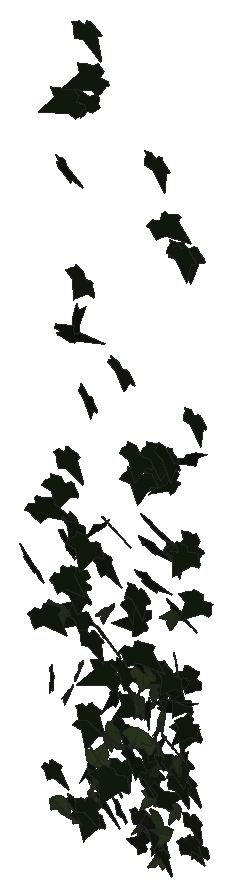
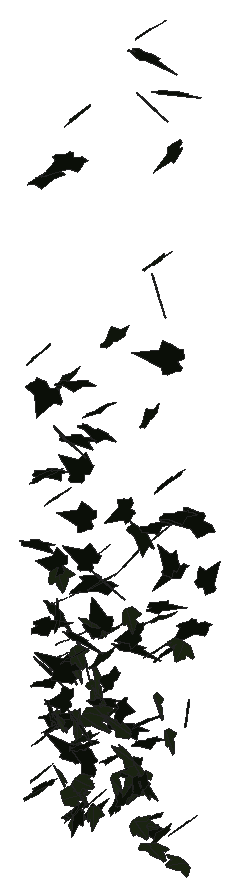
# SketchUp Ruby script. Lengths in inches.
U = 1.inch
M = Sketchup.active_model
def pt(a) = Geom::Point3d.new(a.map { |v| v * U })
def face(e, loops, mat)
  f = e.add_face(loops[0].map { |a| pt(a) })
  loops[1..].each { |l| e.add_face(l.map { |a| pt(a) }).erase! }
  f.material = f.back_material = mat if mat
  f
end
# faces: each face lists its corners as indices into pts; further lists are holes
def faces(e, pts, list, mat = nil) = list.each { |f| face(e, (f[0].is_a?(Array) ? f : [f]).map { |l| l.map { |i| pts[i] } }, mat) }
# xy, xz, yz: faces in a plane at the given z, y or x. An outline is a flat list of corners, or four numbers for a rectangle; further outlines are holes
def ring(l) = l.size == 4 ? [[l[0], l[1]], [l[2], l[1]], [l[2], l[3]], [l[0], l[3]]] : l.each_slice(2).to_a
def flat(e, list, mat, &to3) = list.each { |f| face(e, (f[0].is_a?(Array) ? f : [f]).map { |l| ring(l).map { |u, v| to3.(u, v) } }, mat) }
def xy(e, z, list, mat = nil) = flat(e, list, mat) { |x, y| [x, y, z] }
def xz(e, y, list, mat = nil) = flat(e, list, mat) { |x, z| [x, y, z] }
def yz(e, x, list, mat = nil) = flat(e, list, mat) { |y, z| [x, y, z] }
def lines(e, pts, list) = list.each { |a, b| e.add_line(pt(pts[a]), pt(pts[b])) }
# prism: a flat outline (further loops are holes) pulled along v
def prism(e, loops, v, mat = nil)
  f = face(e, loops, mat); d = Geom::Vector3d.new(v.map { |x| x * U })
  f.pushpull(f.normal.samedirection?(d) ? d.length : -d.length)
end
def box(e, o, s, mat = nil) = prism(e, [[o, [o[0] + s[0], o[1], o[2]], [o[0] + s[0], o[1] + s[1], o[2]], [o[0], o[1] + s[1], o[2]]]], [0, 0, s[2]], mat)
def at(x, y, z, deg = 0) = Geom::Transformation.translation(pt([x, y, z])) * Geom::Transformation.rotation(ORIGIN, Z_AXIS, deg.degrees)
def axes(o, x, y, z) = Geom::Transformation.new([*x, 0, *y, 0, *z, 0, *pt(o).to_a, 1])
def part(name) = M.definitions.add(name)
# library, detail: a bought-in or finely detailed component or shape, given as its bounding box
def library(name, o, s) = part(name).tap { |d| box(d.entities, o, s) }
def detail(e, o, s) = box(e.add_group.entities, o, s)
def put(e, d, t, mat = nil) = e.add_instance(d, t).tap { |i| i.material = mat if mat }
def group(e, t, mat = nil) = e.add_group.tap { |g| g.transformation = t; g.material = mat if mat }.entities
root = M.entities
M.materials.add("1026 AP 7946 SUNNY SIDE UP").color = [254, 231, 186]
M.materials.add("efeu1").color = [18, 25, 13]
M.materials.add("efeu2").color = [43, 57, 29]
c1 = part("ivyleaf_9")
p = [[1.54,2.16,1.25],[1.36,2.04,1.19],[-0.21,0.99,0.68],[-0.71,1.11,0.82],[-0.85,0.86,0.67],[-0.8,0.17,0.21],
  [-0.9,-0.01,0.1],[-0.67,-0.16,-0.02],[-0.08,-0.08,-0.05],[-0.03,-0.6,-0.4],[0.65,-0.88,-0.66],[0.83,-0.6,-0.49],
  [1.29,-0.42,-0.43],[1.8125,-0.07,-0.26],[1.21,0.44,0.15]]
faces(c1.entities,p,[[0,1,2,3,4,5,6,7,8,9,10,11,12,13,14]],"efeu1")
c2 = part("ivyleaf_10")
p = [[0,0.5,-0.03],[-0.0625,2.02,-0.43],[-0.19,2.01,-0.46],[-0.54,1.05,-0.29],[-0.52,0.625,-0.18],[-0.83,0.76,-0.28],
  [-1.16,0.64,-0.33],[-1.15,0.33,-0.24],[-0.77,-0.39,0.02],[-0.3,-0.51,0.16],[0.04,-0.48,0.23],[-0.02,2.01,-0.4375],
  [-0.06,2.01,-0.43],[0.04,-0.49,0.23],[0.67,-0.49,0.14],[1.38,0.36,-0.2],[1.375,0.51,-0.24],[0.81,0.65,-0.19],
  [0.62,0.59,-0.15],[0.6,1.09,-0.28],[0.5,1.23,-0.31]]
faces(c2.entities,p,[[0,1,2,3,4,5,6,7,8,9,10],[11,12,0,13,14,15,16,17,18,19,20]],"efeu2")
put(root,c1,axes([120.64,210.23,304.1],[0.28592,-0.32766,0.26056],[-0.14021,0.24083,0.38604],[-0.63741,-0.19995,0.03197]),"1026 AP 7946 SUNNY SIDE UP")
put(root,c1,axes([120.27,211.82,293.3125],[0.25007,-0.29162,-0.18402],[-0.05716,0.17966,-0.3376],[0.53333,0.156,0.0501]),"1026 AP 7946 SUNNY SIDE UP")
put(root,c2,axes([120.37,212.17,291.41],[-0.39726,-0.00522,-0.27921],[0.39286,-0.14811,-0.23789],[-0.16523,-0.3396,0.10568]),"1026 AP 7946 SUNNY SIDE UP")
put(root,c2,axes([120.76,211.63,301.71],[-0.60127,0.08137,-0.06025],[0.07732,-0.05071,-0.40105],[-0.13777,-0.38357,0.03786]),"1026 AP 7946 SUNNY SIDE UP")
put(root,c1,axes([120.63,211.45,298.32],[0.06531,-0.1363,-0.39031],[0.50627,-0.21622,0.11547],[-0.37825,-0.31294,0.08717]),"1026 AP 7946 SUNNY SIDE UP")
put(root,c2,axes([121.14,212.1,297.37],[0.09032,-0.38326,0.01758],[-0.00117,-0.01956,-0.39934],[0.6034,0.05733,-0.0034]),"1026 AP 7946 SUNNY SIDE UP")
put(root,c1,axes([120.64,210.47,307.37],[0.1737,-0.02062,-0.4547],[0.41121,0.36963,0.05181],[0.55979,-0.26512,0.10303]),"1026 AP 7946 SUNNY SIDE UP")
put(root,c1,axes([121.11,211.67,308.05],[-0.33308,-0.3602,-0.01481],[0.02704,0.00418,-0.43026],[0.56606,-0.21215,0.01184]),"1026 AP 7946 SUNNY SIDE UP")
put(root,c1,axes([120.99,210.36,302.12],[0.04492,-0.24383,-0.39442],[0.00693,0.38237,-0.2492],[0.71187,0.01167,0.02732]),"1026 AP 7946 SUNNY SIDE UP")
put(root,c1,axes([121.37,212.29,301.29],[-0.17419,-0.264,0.2771],[-0.14262,-0.25505,-0.29622],[0.57695,-0.14276,0.01044]),"1026 AP 7946 SUNNY SIDE UP")
put(root,c1,axes([121.31,211.56,309.73],[0.22359,-0.39067,-0.18284],[-0.06426,0.17145,-0.42686],[0.6702,0.14677,0.02007]),"1026 AP 7946 SUNNY SIDE UP")
put(root,c1,axes([120.99,211.83,315.69],[0.4611,-0.03933,0.35691],[0.54226,-0.03601,-0.30494],[0.08321,0.45264,0.00944]),"1026 AP 7946 SUNNY SIDE UP")
put(root,c1,axes([122.03,211.96,303.28],[-0.37134,-0.08589,0.31608],[-0.40952,-0.169,-0.25583],[0.28987,-0.34878,0.04348]),"1026 AP 7946 SUNNY SIDE UP")
put(root,c2,axes([121.82,212,298.82],[0.17687,-0.3738,-0.04632],[-0.03405,0.03821,-0.4018],[0.59064,0.11414,-0.00929]),"1026 AP 7946 SUNNY SIDE UP")
put(root,c1,axes([121.38,211.51,305.21],[0.11465,-0.13289,0.42396],[0.22216,-0.38793,-0.15682],[0.64387,0.15751,-0.02138]),"1026 AP 7946 SUNNY SIDE UP")
put(root,c1,axes([122.14,211.12,328.17],[-0.65585,-0.11577,0.19889],[-0.20333,-0.21101,-0.41799],[0.29082,-0.40862,0.15628]),"1026 AP 7946 SUNNY SIDE UP")
put(root,c1,axes([121.7,212.22,301.41],[-0.04768,-0.38202,0.08659],[0.00998,-0.08694,-0.39508],[0.61572,-0.02817,0.01311]),"1026 AP 7946 SUNNY SIDE UP")
put(root,c2,axes([122.04,212.1,291.61],[0.54998,0.07879,-0.16507],[-0.22999,-0.07736,-0.36756],[-0.16212,0.37706,-0.03853]),"1026 AP 7946 SUNNY SIDE UP")
put(root,c1,axes([121.8,211.83,302.75],[-0.15081,-0.36461,0.12107],[0.10561,-0.13732,-0.37662],[0.59406,-0.06815,0.09769]),"1026 AP 7946 SUNNY SIDE UP")
put(root,c1,axes([122.42,211.65,327.63],[0.03759,0.28344,0.38774],[-0.34589,0.33834,-0.24718],[-0.65288,-0.16293,0.15328]),"1026 AP 7946 SUNNY SIDE UP")
put(root,c1,axes([121.82,211.69,292.02],[0.07471,-0.33256,0.17753],[0.04916,-0.17149,-0.34702],[0.58827,0.05656,0.00645]),"1026 AP 7946 SUNNY SIDE UP")
put(root,c1,axes([121.91,210.5,325.17],[0.55052,-0.19879,-0.24116],[-0.25395,0.18079,-0.40792],[0.40915,0.3797,0.0713]),"1026 AP 7946 SUNNY SIDE UP")
put(root,c1,axes([122.21,211.28,306.54],[-0.11855,-0.3498,0.27052],[-0.07175,-0.26074,-0.37007],[0.6859,-0.08773,0.00804]),"1026 AP 7946 SUNNY SIDE UP")
put(root,c1,axes([122.07,212.21,312.61],[0.05601,-0.32266,0.29324],[0.03549,-0.28567,-0.33603],[0.67755,0.04164,-0.00664]),"1026 AP 7946 SUNNY SIDE UP")
put(root,c1,axes([122.15,210.25,304.42],[0.1826,-0.23016,-0.39573],[-0.15822,0.3719,-0.25961],[0.68431,0.1474,0.04557]),"1026 AP 7946 SUNNY SIDE UP")
put(root,c1,axes([122.17,211.89,331.63],[0.16087,-0.46178,-0.08563],[0.02278,0.08547,-0.48563],[0.7367,0.09819,0.03372]),"1026 AP 7946 SUNNY SIDE UP")
put(root,c2,axes([122.82,212.02,292.36],[-0.13485,-0.08859,0.3881],[-0.12572,-0.374,-0.11139],[0.59618,-0.0989,0.06429]),"1026 AP 7946 SUNNY SIDE UP")
put(root,c1,axes([122.76,211.85,294.38],[-0.41219,0.13402,-0.25345],[0.28629,-0.17592,-0.29869],[-0.3362,-0.31412,0.05639]),"1026 AP 7946 SUNNY SIDE UP")
put(root,c2,axes([122.8,212.14,292.47],[-0.14475,-0.32546,0.16154],[-0.06372,-0.15341,-0.34933],[0.56574,-0.10055,0.00199]),"1026 AP 7946 SUNNY SIDE UP")
put(root,c1,axes([122.72,211.67,296.36],[-0.26108,-0.34409,0.01151],[0.00965,-0.01753,-0.39347],[0.54136,-0.16563,0.01256]),"1026 AP 7946 SUNNY SIDE UP")
put(root,c1,axes([122.59,210.66,317.19],[-0.08631,0.29408,0.38045],[0.0137,-0.36943,0.30362],[0.74014,0.04113,0.03874]),"1026 AP 7946 SUNNY SIDE UP")
put(root,c1,axes([122.47,212.27,294.43],[0.10747,-0.21577,0.30857],[0.15015,-0.28521,-0.23482],[0.56232,0.1174,0.00373]),"1026 AP 7946 SUNNY SIDE UP")
put(root,c1,axes([123.03,211.56,306.38],[0.05282,0.35942,0.20714],[-0.07175,0.20172,-0.36617],[-0.64202,0.00702,0.05796]),"1026 AP 7946 SUNNY SIDE UP")
put(root,c1,axes([122.67,211.36,292.52],[0.05375,-0.34473,-0.13537],[0.06115,0.13266,-0.35259],[0.57577,0.01809,0.05009]),"1026 AP 7946 SUNNY SIDE UP")
put(root,c1,axes([123.39,211.29,329.72],[-0.72598,0.01031,0.131],[-0.2005,-0.03122,-0.47474],[-0.00257,-0.47786,0.03103]),"1026 AP 7946 SUNNY SIDE UP")
put(root,c1,axes([122.85,210.95,319.41],[-0.20814,-0.34151,0.31042],[-0.03857,-0.30997,-0.37245],[0.71711,-0.11579,0.07006]),"1026 AP 7946 SUNNY SIDE UP")
put(root,c1,axes([122.95,211.34,291.93],[-0.41786,-0.2819,-0.06938],[0.09697,0.03206,-0.39824],[0.4447,-0.27188,0.02165]),"1026 AP 7946 SUNNY SIDE UP")
put(root,c1,axes([122.73,211.37,297.3],[0.11506,-0.35302,-0.13854],[0.06617,0.14175,-0.36437],[0.58919,0.05302,0.06797]),"1026 AP 7946 SUNNY SIDE UP")
put(root,c2,axes([123,211.6875,294.6],[0.58621,0.07165,-0.11698],[0.16344,0.06,0.38952],[0.1345,-0.3852,0.03653]),"1026 AP 7946 SUNNY SIDE UP")
put(root,c1,axes([122.97,211.73,293.71],[0.05927,-0.35137,0.12483],[0.04024,-0.12106,-0.36456],[0.58408,0.044,0.01245]),"1026 AP 7946 SUNNY SIDE UP")
put(root,c2,axes([123.27,211.2,293.98],[0.35127,-0.27592,0.12698],[0.09389,-0.11195,-0.36565],[0.46685,0.23013,-0.02201]),"1026 AP 7946 SUNNY SIDE UP")
put(root,c1,axes([123.34,210.68,306.24],[-0.32115,-0.39941,0.04033],[-0.00342,-0.04536,-0.46201],[0.63139,-0.2034,0.01801]),"1026 AP 7946 SUNNY SIDE UP")
put(root,c2,axes([123.48,211.875,302.43],[-0.07683,-0.40129,0.00616],[-0.00089,-0.00825,-0.41651],[0.63112,-0.04886,0.00016]),"1026 AP 7946 SUNNY SIDE UP")
put(root,c2,axes([123.25,211.66,293.75],[0.29355,0.32363,0.10241],[0.09777,0.07668,-0.38414],[-0.52244,0.1962,-0.01435]),"1026 AP 7946 SUNNY SIDE UP")
put(root,c2,axes([123.51,211.98,294.01],[0.011,0.17683,-0.36811],[-0.18391,-0.34178,-0.17811],[-0.60079,0.10786,0.04778]),"1026 AP 7946 SUNNY SIDE UP")
put(root,c1,axes([123.21,211.59,301.39],[0.47886,-0.28718,0.05838],[0.04073,-0.05736,-0.43087],[0.45896,0.30472,-0.02267]),"1026 AP 7946 SUNNY SIDE UP")
put(root,c1,axes([123.57,212.36,297.93],[-0.09674,-0.02371,-0.38608],[0.33345,-0.31545,-0.01715],[-0.48704,-0.21126,0.06494]),"1026 AP 7946 SUNNY SIDE UP")
put(root,c1,axes([123.28,212.3,293.64],[0.17645,-0.2851,0.21587],[0.11909,-0.19711,-0.31679],[0.545,0.13537,-0.00067]),"1026 AP 7946 SUNNY SIDE UP")
put(root,c2,axes([123.22,212.24,295.62],[-0.04957,-0.03332,-0.40747],[0.48725,-0.24972,-0.00523],[-0.38957,-0.3081,0.0453]),"1026 AP 7946 SUNNY SIDE UP")
put(root,c1,axes([123.38,210.74,301.53],[0.12962,-0.38118,-0.07742],[0.01883,0.07708,-0.40031],[0.60996,0.07862,0.02881]),"1026 AP 7946 SUNNY SIDE UP")
put(root,c1,axes([123.46,211.46,305.14],[0.36664,-0.32796,-0.23384],[-0.1819,0.19377,-0.4131],[0.59845,0.25982,0.0177]),"1026 AP 7946 SUNNY SIDE UP")
put(root,c2,axes([124.03,212.15,294.14],[0.16663,-0.29247,0.2232],[0.108,-0.20729,-0.32164],[0.56362,0.12618,-0.00435]),"1026 AP 7946 SUNNY SIDE UP")
put(root,c1,axes([123.86,211.36,307.2],[0.57223,-0.19088,-0.04524],[-0.05277,0.02821,-0.42307],[0.30305,0.36534,0.01177]),"1026 AP 7946 SUNNY SIDE UP")
put(root,c1,axes([124.62,210.78,299.99],[-0.67335,-0.05968,0.16477],[-0.23459,-0.08095,-0.44216],[0.1315,-0.45002,0.05492]),"1026 AP 7946 SUNNY SIDE UP")
put(root,c2,axes([123.87,211.68,296.48],[0.14124,-0.07392,-0.39609],[0.55906,-0.14875,0.11429],[-0.25623,-0.3653,0.03103]),"1026 AP 7946 SUNNY SIDE UP")
put(root,c1,axes([124.3,211.77,292.48],[-0.1354,-0.09739,0.35367],[0.01047,-0.35408,-0.10367],[0.56186,-0.01688,0.08716]),"1026 AP 7946 SUNNY SIDE UP")
put(root,c1,axes([124.22,212.05,298.91],[0.26532,-0.30259,0.17383],[0.09838,-0.15992,-0.35721],[0.53716,0.17875,-0.02044]),"1026 AP 7946 SUNNY SIDE UP")
put(root,c1,axes([124.86,212.27,297.85],[-0.50579,-0.1734,0.13073],[-0.14932,-0.09216,-0.37536],[0.30411,-0.33366,0.03312]),"1026 AP 7946 SUNNY SIDE UP")
put(root,c1,axes([124.49,211.58,294.97],[0.00688,-0.38292,-0.0576],[0.02187,0.05386,-0.39391],[0.60761,0.0024,0.01483]),"1026 AP 7946 SUNNY SIDE UP")
put(root,c1,axes([124.41,210.23,293.76],[0.41446,-0.32861,0.04046],[0.00754,-0.04879,-0.4334],[0.52069,0.26227,-0.02593]),"1026 AP 7946 SUNNY SIDE UP")
put(root,c1,axes([124.64,211.59,297],[-0.00867,-0.35213,0.15957],[0.02357,-0.15699,-0.36335],[0.6057,0.00107,0.01642]),"1026 AP 7946 SUNNY SIDE UP")
put(root,c1,axes([124.64,211.42,315.26],[-0.06484,-0.36348,0.30194],[0.12179,-0.29751,-0.36803],[0.72609,0.01744,0.0887]),"1026 AP 7946 SUNNY SIDE UP")
put(root,c2,axes([125.01,212.18,298.16],[0.47222,-0.23025,0.08832],[0.0832,-0.0737,-0.38939],[0.378,0.30386,-0.02463]),"1026 AP 7946 SUNNY SIDE UP")
put(root,c2,axes([125.16,212.01,298.29],[-0.49597,0.2392,-0.00275],[-0.02631,-0.0287,-0.40657],[-0.37525,-0.31414,0.03214]),"1026 AP 7946 SUNNY SIDE UP")
put(root,c2,axes([125.23,211.98,298.97],[0.13471,-0.34509,-0.18866],[-0.06086,0.17705,-0.36524],[0.60983,0.0939,0.00523]),"1026 AP 7946 SUNNY SIDE UP")
put(root,c2,axes([125.37,211.9,292.07],[-0.06168,-0.37464,-0.10863],[0.05387,0.10011,-0.38676],[0.60869,-0.04682,0.02322]),"1026 AP 7946 SUNNY SIDE UP")
put(root,c1,axes([125.42,209.94,295.39],[-0.55363,-0.30265,-0.02997],[0.0644,-0.00575,-0.47728],[0.47348,-0.35311,0.02987]),"1026 AP 7946 SUNNY SIDE UP")
put(root,c1,axes([125.2,211.66,303.24],[-0.07413,-0.37507,0.14546],[0.03902,-0.14675,-0.38809],[0.63014,-0.03504,0.04114]),"1026 AP 7946 SUNNY SIDE UP")
put(root,c2,axes([125.71,211.83,296.5],[0.37607,-0.02662,-0.32091],[-0.49119,-0.03076,-0.24467],[-0.01303,0.3914,-0.03874]),"1026 AP 7946 SUNNY SIDE UP")
put(root,c2,axes([125.47,211.55,296.91],[0.48073,0.18326,-0.17949],[-0.20594,-0.12097,-0.36637],[-0.34143,0.33099,-0.03173]),"1026 AP 7946 SUNNY SIDE UP")
put(root,c1,axes([125.29,210.91,300.44],[-0.09389,-0.34347,0.18712],[0.03158,-0.1882,-0.3571],[0.61157,-0.04301,0.04717]),"1026 AP 7946 SUNNY SIDE UP")
put(root,c1,axes([125.34,211.8,292.69],[0.20542,-0.3735,-0.09907],[-0.05676,0.087,-0.40709],[0.60296,0.13544,-0.00457]),"1026 AP 7946 SUNNY SIDE UP")
put(root,c2,axes([125.64,210.89,296.63],[0.25166,-0.3255,0.1427],[0.07931,-0.13154,-0.37424],[0.55172,0.16738,-0.01129]),"1026 AP 7946 SUNNY SIDE UP")
put(root,c1,axes([126.27,210.91,303.15],[-0.54594,0.28765,0.14026],[-0.21222,0.04674,-0.46157],[-0.45197,-0.3694,0.04731]),"1026 AP 7946 SUNNY SIDE UP")
put(root,c2,axes([125.85,212.26,293.54],[-0.17868,-0.19282,0.32316],[-0.01723,-0.32746,-0.21263],[0.5802,-0.06911,0.09321]),"1026 AP 7946 SUNNY SIDE UP")
put(root,c1,axes([125.89,211.47,291.48],[-0.04544,0.00008,0.38116],[-0.36441,-0.28929,-0.02027],[0.4535,-0.23246,0.0219]),"1026 AP 7946 SUNNY SIDE UP")
put(root,c1,axes([125.75,212.23,295.57],[-0.23672,-0.27142,0.22185],[0.04935,-0.24604,-0.29619],[0.54408,-0.09578,0.12339]),"1026 AP 7946 SUNNY SIDE UP")
put(root,c1,axes([125.71,211.29,311.38],[-0.17289,-0.43324,0.11697],[-0.01147,-0.1177,-0.46065],[0.70514,-0.10814,0.02119]),"1026 AP 7946 SUNNY SIDE UP")
put(root,c1,axes([125.34,212.16,304.44],[0.25728,-0.16076,0.34211],[0.40001,-0.21532,-0.23713],[0.42196,0.30214,0.0162]),"1026 AP 7946 SUNNY SIDE UP")
put(root,c1,axes([125.66,211.28,304.33],[0.03322,-0.40855,0.07382],[0.00634,-0.07386,-0.42188],[0.65282,0.02151,0.00034]),"1026 AP 7946 SUNNY SIDE UP")
put(root,c1,axes([125.42,211.98,294.45],[0.33199,-0.07389,-0.35273],[0.5501,0.04011,0.21382],[-0.00617,-0.39989,0.08418]),"1026 AP 7946 SUNNY SIDE UP")
put(root,c1,axes([125.56,211.12,300.63],[0.62746,-0.15796,-0.14405],[0.22647,-0.01198,0.44015],[-0.24108,-0.42237,0.03856]),"1026 AP 7946 SUNNY SIDE UP")
put(root,c1,axes([125.875,211.25,310.34],[-0.4839,-0.2086,-0.20936],[0.32613,0.04817,-0.37641],[0.31962,-0.36497,0.06711]),"1026 AP 7946 SUNNY SIDE UP")
put(root,c1,axes([125.89,211.85,295.79],[-0.18535,0.33808,0.15869],[0.08747,-0.14168,0.36798],[0.57633,0.13023,-0.00482]),"1026 AP 7946 SUNNY SIDE UP")
put(root,c1,axes([125.53,212.06,306.39],[0.435,-0.17323,0.25518],[0.33292,-0.13046,-0.33702],[0.34098,0.34837,0.00351]),"1026 AP 7946 SUNNY SIDE UP")
put(root,c1,axes([125.99,211.78,295.08],[-0.07497,-0.36936,-0.05972],[0.04417,0.05262,-0.38276],[0.58573,-0.05124,0.02122]),"1026 AP 7946 SUNNY SIDE UP")
put(root,c1,axes([126.31,212.22,310.24],[-0.54541,-0.23146,0.03732],[-0.01904,-0.04925,-0.42844],[0.36822,-0.34539,0.03312]),"1026 AP 7946 SUNNY SIDE UP")
put(root,c1,axes([126.3,211.78,291.66],[-0.00486,-0.04522,-0.39564],[-0.41324,0.28163,-0.03036],[0.44549,0.26074,-0.03248]),"1026 AP 7946 SUNNY SIDE UP")
put(root,c2,axes([126.25,211.9375,296.46],[-0.38456,0.29549,0.07603],[-0.10268,0.03938,-0.3941],[-0.46711,-0.25192,0.02404]),"1026 AP 7946 SUNNY SIDE UP")
put(root,c2,axes([126.45,211.71,292.82],[0.29782,-0.18902,-0.29254],[-0.31346,0.20072,-0.27449],[0.43353,0.27498,0.0025]),"1026 AP 7946 SUNNY SIDE UP")
put(root,c2,axes([126.29,211.97,299.58],[-0.07839,-0.38194,0.11222],[0.00572,-0.1124,-0.39706],[0.62543,-0.04684,0.0177]),"1026 AP 7946 SUNNY SIDE UP")
put(root,c1,axes([126.61,211.875,300.3],[-0.61328,0.05098,0.09296],[-0.14715,-0.02489,-0.40368],[-0.06909,-0.39949,0.03463]),"1026 AP 7946 SUNNY SIDE UP")
put(root,c1,axes([126.03,212.11,326.09],[0.1233,-0.45814,0.07365],[0.00146,-0.07498,-0.47913],[0.72974,0.07756,-0.01148]),"1026 AP 7946 SUNNY SIDE UP")
put(root,c1,axes([126.05,212.17,291.99],[0.20541,-0.34434,0.02961],[-0.00062,-0.03296,-0.3794],[0.54359,0.13008,-0.01162]),"1026 AP 7946 SUNNY SIDE UP")
put(root,c2,axes([126.14,211.01,300.54],[0.60018,-0.05138,0.10117],[0.14489,-0.05045,-0.39527],[0.09757,0.39096,-0.03535]),"1026 AP 7946 SUNNY SIDE UP")
put(root,c1,axes([126.06,211.47,298.61],[-0.08502,-0.09294,-0.41061],[0.59216,-0.16742,-0.01341],[-0.24987,-0.36515,0.10793]),"1026 AP 7946 SUNNY SIDE UP")
put(root,c1,axes([126.2,212.1875,299.57],[-0.0153,-0.3942,0.01935],[0.00182,-0.02106,-0.40634],[0.62071,-0.00966,0.00167]),"1026 AP 7946 SUNNY SIDE UP")
put(root,c1,axes([126.23,211.67,292.49],[0.00081,-0.37565,0.15117],[-0.01104,-0.14886,-0.3878],[0.63527,-0.00211,-0.00693]),"1026 AP 7946 SUNNY SIDE UP")
put(root,c2,axes([126.52,211.58,295.62],[0.04287,-0.35967,-0.1321],[0.0111,0.12696,-0.3705],[0.59923,0.02338,0.01632]),"1026 AP 7946 SUNNY SIDE UP")
put(root,c2,axes([126.88,211.76,292.16],[-0.09986,-0.08441,-0.38653],[-0.44809,-0.24431,0.10502],[-0.40497,0.29114,-0.02089]),"1026 AP 7946 SUNNY SIDE UP")
put(root,c2,axes([126.68,211.23,299.42],[0.29008,-0.33447,-0.09941],[-0.02547,0.09871,-0.3915],[0.54596,0.18232,0.03456]),"1026 AP 7946 SUNNY SIDE UP")
put(root,c1,axes([126.76,212.13,300.07],[-0.34176,-0.17962,0.28665],[-0.14378,-0.28849,-0.26616],[0.50192,-0.20495,0.11894]),"1026 AP 7946 SUNNY SIDE UP")
put(root,c2,axes([126.73,211.58,291.08],[0.05767,0.12037,-0.37807],[-0.17798,-0.34982,-0.13166],[-0.5817,0.11897,0.0028]),"1026 AP 7946 SUNNY SIDE UP")
put(root,c1,axes([127.09,212.08,310.15],[-0.58856,0.18382,-0.05959],[0.0506,-0.06725,-0.4274],[-0.29926,-0.37289,0.04493]),"1026 AP 7946 SUNNY SIDE UP")
put(root,c1,axes([126.42,210.11,302.2],[0.04232,-0.19811,-0.41305],[0.24353,0.37979,-0.1809],[0.658,-0.12782,0.09352]),"1026 AP 7946 SUNNY SIDE UP")
put(root,c1,axes([126.66,211.57,296.05],[0.43665,-0.25353,-0.09169],[-0.0467,0.0962,-0.38342],[0.41916,0.27483,0.0528]),"1026 AP 7946 SUNNY SIDE UP")
put(root,c1,axes([126.7,211.56,291.42],[0.22744,-0.34182,0.02511],[-0.00402,-0.02964,-0.38228],[0.53905,0.144,-0.01345]),"1026 AP 7946 SUNNY SIDE UP")
put(root,c2,axes([127.08,212.17,303.28],[-0.2574,-0.36372,0.06428],[0.00268,-0.07125,-0.41013],[0.58082,-0.16086,0.03038]),"1026 AP 7946 SUNNY SIDE UP")
put(root,c1,axes([126.51,211.23,308],[0.23352,-0.25521,0.3576],[0.35049,-0.27047,-0.30343],[0.58189,0.26533,0.03926]),"1026 AP 7946 SUNNY SIDE UP")
put(root,c1,axes([126.59,211.95,298.57],[0.40268,0.25342,-0.2107],[0.19793,0.16491,0.37125],[0.47381,-0.28427,0.02398]),"1026 AP 7946 SUNNY SIDE UP")
put(root,c2,axes([126.85,211.57,298.3],[0.32452,-0.22806,0.26871],[0.28438,-0.18981,-0.31794],[0.46649,0.27437,0.00689]),"1026 AP 7946 SUNNY SIDE UP")
put(root,c1,axes([126.8,211.59,323.48],[0.08857,-0.19072,-0.43811],[0.03537,0.4279,-0.19262],[0.73045,0.00241,0.06245]),"1026 AP 7946 SUNNY SIDE UP")
put(root,c1,axes([126.7,211.39,294.09],[-0.03963,0.05626,0.4025],[0.57083,-0.14962,0.04548],[0.24245,0.36145,-0.04129]),"1026 AP 7946 SUNNY SIDE UP")
put(root,c2,axes([127.17,210.89,298.13],[0.17136,-0.37127,0.04369],[0.00206,-0.04599,-0.3987],[0.58796,0.10837,-0.01134]),"1026 AP 7946 SUNNY SIDE UP")
put(root,c2,axes([127.21,212.04,293.46],[0.44081,-0.23029,0.02573],[0.0025,-0.03934,-0.37276],[0.36445,0.27881,-0.02857]),"1026 AP 7946 SUNNY SIDE UP")
put(root,c2,axes([127.25,211.91,296],[0.24001,-0.33701,0.1398],[0.04898,-0.13658,-0.38097],[0.57029,0.15356,-0.02612]),"1026 AP 7946 SUNNY SIDE UP")
put(root,c1,axes([126.86,211.8,296.97],[0.46095,-0.25999,0.09646],[0.07816,-0.08685,-0.4029],[0.42823,0.29571,-0.0303]),"1026 AP 7946 SUNNY SIDE UP")
put(root,c1,axes([127.17,211.06,312.13],[-0.31772,-0.36936,-0.09076],[0.15678,0.04228,-0.42815],[0.57534,-0.21549,0.06655]),"1026 AP 7946 SUNNY SIDE UP")
put(root,c1,axes([127.41,212.32,298.96],[-0.25478,-0.29242,0.19926],[-0.0188,-0.2101,-0.3359],[0.55241,-0.14202,0.08047]),"1026 AP 7946 SUNNY SIDE UP")
put(root,c1,axes([127.28,212.05,300.6],[-0.02075,-0.01426,0.43103],[-0.02626,-0.41833,-0.01767],[0.65787,-0.01715,0.01289]),"1026 AP 7946 SUNNY SIDE UP")
put(root,c1,axes([127.03,212.09,303.64],[0.41681,-0.24083,0.21503],[0.19719,-0.17268,-0.36794],[0.46223,0.29084,-0.03693]),"1026 AP 7946 SUNNY SIDE UP")
put(root,c1,axes([127.33,208.97,297.47],[-0.04046,-0.35317,0.25146],[0.05666,-0.24744,-0.36338],[0.67447,-0.0004,0.04561]),"1026 AP 7946 SUNNY SIDE UP")
put(root,c1,axes([127.73,211.75,296.01],[0.05177,0.12488,0.3721],[-0.01436,0.36198,-0.12621],[-0.5997,0.00211,0.03514]),"1026 AP 7946 SUNNY SIDE UP")
put(root,c1,axes([127.4,211.88,296.07],[-0.17413,-0.34818,-0.15586],[0.13476,0.1285,-0.37344],[0.58026,-0.13433,0.03996]),"1026 AP 7946 SUNNY SIDE UP")
put(root,c1,axes([127.42,211.82,306.75],[0.00161,-0.39552,0.1115],[0.02175,-0.11038,-0.40789],[0.64536,0.00471,0.01347]),"1026 AP 7946 SUNNY SIDE UP")
put(root,c2,axes([127.76,211.48,295.95],[0.07667,0.132,-0.3813],[-0.05568,0.37366,0.1344],[0.61648,0.01733,0.05956]),"1026 AP 7946 SUNNY SIDE UP")
put(root,c1,axes([127.55,211.07,312.06],[0.02579,-0.41045,0.22831],[0.02778,-0.22338,-0.42442],[0.73469,0.02286,0.00803]),"1026 AP 7946 SUNNY SIDE UP")
put(root,c1,axes([128.11,212.21,300.36],[-0.15666,-0.23508,-0.31979],[-0.06217,-0.31129,0.25522],[-0.60743,0.09249,0.05635]),"1026 AP 7946 SUNNY SIDE UP")
put(root,c1,axes([127.875,212.2,297.7],[-0.29906,-0.32863,0.05693],[-0.01453,-0.06055,-0.39086],[0.52429,-0.18914,0.02164]),"1026 AP 7946 SUNNY SIDE UP")
put(root,c1,axes([127.74,211.53,295.32],[0.09377,-0.37275,-0.07251],[0.00199,0.0693,-0.38829],[0.59586,0.05843,0.01271]),"1026 AP 7946 SUNNY SIDE UP")
put(root,c1,axes([128,211.73,311.78],[0.30902,0.39014,0.06742],[0.06503,0.04992,-0.44949],[-0.61804,0.20032,-0.01359]),"1026 AP 7946 SUNNY SIDE UP")
put(root,c1,axes([127.78,212.07,295.09],[0.23278,-0.33711,-0.09396],[-0.04157,0.08588,-0.37865],[0.54677,0.15005,0.01122]),"1026 AP 7946 SUNNY SIDE UP")
put(root,c1,axes([128.02,210.79,301.05],[-0.26425,-0.30234,0.21134],[-0.03542,-0.21863,-0.34932],[0.57494,-0.15243,0.07561]),"1026 AP 7946 SUNNY SIDE UP")
put(root,c1,axes([128.27,211.8,298.23],[-0.61761,0.0594,-0.13961],[0.19949,-0.06446,-0.40729],[-0.12066,-0.41059,0.04123]),"1026 AP 7946 SUNNY SIDE UP")
put(root,c1,axes([128.47,210.83,300.55],[-0.32525,0.33765,0.07397],[-0.09863,0.04329,-0.40647],[-0.53312,-0.214,0.03007]),"1026 AP 7946 SUNNY SIDE UP")
put(root,c1,axes([128.02,211.89,322.28],[-0.13773,-0.44946,-0.06549],[0.02223,0.05941,-0.47139],[0.71287,-0.08869,0.00205]),"1026 AP 7946 SUNNY SIDE UP")
put(root,c1,axes([127.96,212.21,293.17],[0.15772,-0.34947,-0.01219],[-0.00738,0.0089,-0.3745],[0.54967,0.1004,-0.00153]),"1026 AP 7946 SUNNY SIDE UP")
put(root,c1,axes([128.44,211.9375,307.34],[-0.31976,-0.13263,0.3573],[-0.28958,-0.30829,-0.23399],[0.50827,-0.25908,0.09147]),"1026 AP 7946 SUNNY SIDE UP")
put(root,c1,axes([128.03,211.42,322.51],[0.01745,-0.46912,0.08349],[0.00915,-0.08359,-0.48389],[0.74924,0.01195,0.00397]),"1026 AP 7946 SUNNY SIDE UP")
put(root,c1,axes([128.45,212.3,304.37],[-0.5379,-0.20612,0.06215],[-0.05146,-0.06432,-0.40998],[0.33429,-0.34157,0.0369]),"1026 AP 7946 SUNNY SIDE UP")
put(root,c1,axes([128.11,212.24,313.67],[0.08412,-0.41518,0.09625],[-0.00282,-0.09676,-0.43158],[0.66997,0.05172,-0.0139]),"1026 AP 7946 SUNNY SIDE UP")
put(root,c1,axes([128.2,211.62,292.35],[0.17356,-0.29493,-0.21157],[-0.03319,0.20742,-0.31995],[0.56262,0.10322,0.04639]),"1026 AP 7946 SUNNY SIDE UP")
put(root,c1,axes([128.52,211.2,307.35],[-0.43592,-0.30963,0.03678],[-0.0011,-0.04951,-0.42714],[0.49042,-0.27533,0.03174]),"1026 AP 7946 SUNNY SIDE UP")
put(root,c1,axes([128.46,212.25,291.91],[-0.20834,-0.23621,0.25065],[-0.01112,-0.26059,-0.26467],[0.53461,-0.09747,0.09218]),"1026 AP 7946 SUNNY SIDE UP")
